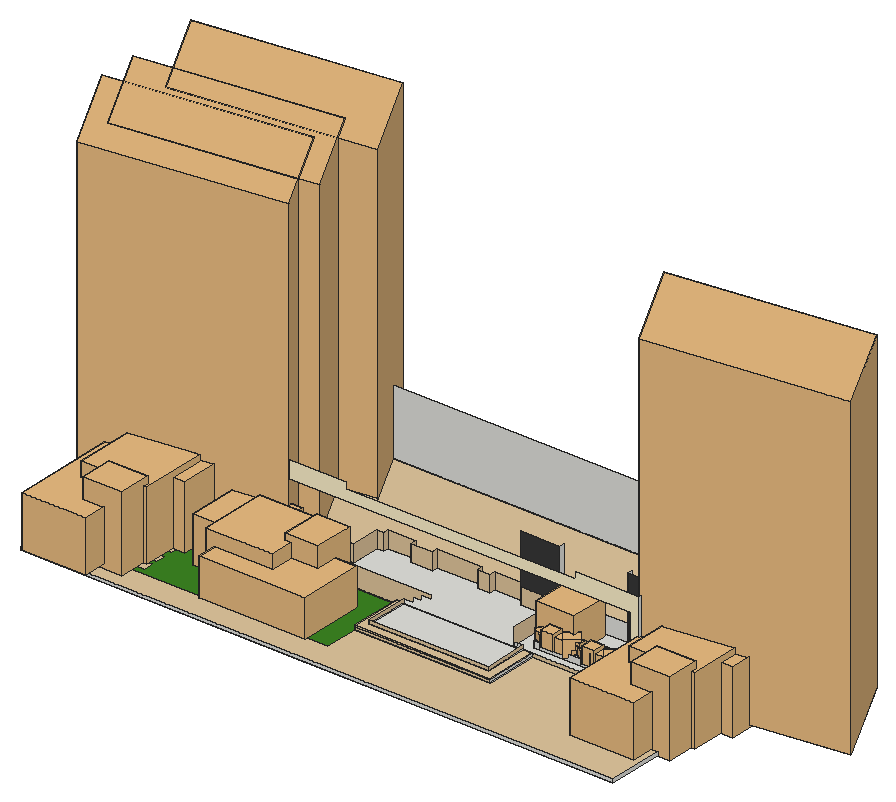
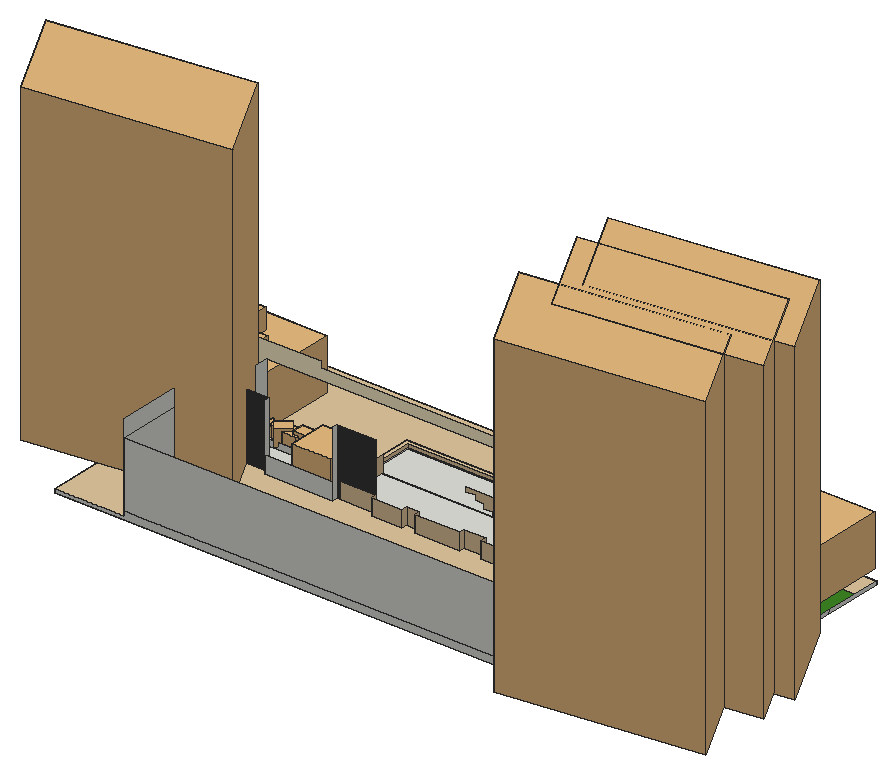
# SketchUp Ruby script. Lengths in inches.
U = 1.inch
M = Sketchup.active_model
def pt(a) = Geom::Point3d.new(a.map { |v| v * U })
def face(e, loops, mat)
  f = e.add_face(loops[0].map { |a| pt(a) })
  loops[1..].each { |l| e.add_face(l.map { |a| pt(a) }).erase! }
  f.material = f.back_material = mat if mat
  f
end
# faces: each face lists its corners as indices into pts; further lists are holes
def faces(e, pts, list, mat = nil) = list.each { |f| face(e, (f[0].is_a?(Array) ? f : [f]).map { |l| l.map { |i| pts[i] } }, mat) }
# xy, xz, yz: faces in a plane at the given z, y or x. An outline is a flat list of corners, or four numbers for a rectangle; further outlines are holes
def ring(l) = l.size == 4 ? [[l[0], l[1]], [l[2], l[1]], [l[2], l[3]], [l[0], l[3]]] : l.each_slice(2).to_a
def flat(e, list, mat, &to3) = list.each { |f| face(e, (f[0].is_a?(Array) ? f : [f]).map { |l| ring(l).map { |u, v| to3.(u, v) } }, mat) }
def xy(e, z, list, mat = nil) = flat(e, list, mat) { |x, y| [x, y, z] }
def xz(e, y, list, mat = nil) = flat(e, list, mat) { |x, z| [x, y, z] }
def yz(e, x, list, mat = nil) = flat(e, list, mat) { |y, z| [x, y, z] }
def lines(e, pts, list) = list.each { |a, b| e.add_line(pt(pts[a]), pt(pts[b])) }
# prism: a flat outline (further loops are holes) pulled along v
def prism(e, loops, v, mat = nil)
  f = face(e, loops, mat); d = Geom::Vector3d.new(v.map { |x| x * U })
  f.pushpull(f.normal.samedirection?(d) ? d.length : -d.length)
end
def box(e, o, s, mat = nil) = prism(e, [[o, [o[0] + s[0], o[1], o[2]], [o[0] + s[0], o[1] + s[1], o[2]], [o[0], o[1] + s[1], o[2]]]], [0, 0, s[2]], mat)
def at(x, y, z, deg = 0) = Geom::Transformation.translation(pt([x, y, z])) * Geom::Transformation.rotation(ORIGIN, Z_AXIS, deg.degrees)
def axes(o, x, y, z) = Geom::Transformation.new([*x, 0, *y, 0, *z, 0, *pt(o).to_a, 1])
def part(name) = M.definitions.add(name)
# library, detail: a bought-in or finely detailed component or shape, given as its bounding box
def library(name, o, s) = part(name).tap { |d| box(d.entities, o, s) }
def detail(e, o, s) = box(e.add_group.entities, o, s)
def put(e, d, t, mat = nil) = e.add_instance(d, t).tap { |i| i.material = mat if mat }
def group(e, t, mat = nil) = e.add_group.tap { |g| g.transformation = t; g.material = mat if mat }.entities
root = M.entities
M.materials.add("Material__1").color = [95, 70, 46]
M.materials.add("[Color A01]").color = [60, 133, 34]
M.materials.add("[Color D01]").color = [255, 242, 204]
M.materials.add("[Color M08]").color = [56, 56, 56]
M.materials.add("[Formica Beige]").color = [226, 199, 158]
c1 = library("Pot+Plant",[-20.81,-17.08,-0.03],[39.86,39.43,41.33])
c2 = library("Potted broadleaf plant",[-29.7,0,-10.87],[31.67,38.52,72.45])
c3 = part("Monstera_Pot_Quarter")
detail(c3.entities,[0.23,0.23,0],[9.32,9.32,13.9])
c4 = part("Monstera_Stem")
p = [[0.53,2.46,1.55],[0.55,2.41,0.71],[0.58,2.34,0.01],[0.58,2.59,0.01],[0.53,2.71,1.56],[0.48,2.66,3.11],
  [0.43,2.45,4.65],[0.38,2.07,6.15],[0.34,1.53,7.61],[0.29,0.84,9],[0.25,0,10.3125],[0.27,0.15,9.7],
  [0.3,0.62,8.89],[0.3,0.62,8.88],[0.34,1.3,7.51],[0.38,1.83,6.08],[0.43,2.2,4.6],[0.48,2.41,3.09],
  [0.53,2.46,1.5625],[0.33,2.59,0],[0.28,2.71,1.55],[0.23,2.66,3.1],[0.18,2.45,4.64],[0.13,2.07,6.15],
  [0.09,1.53,7.6],[0.04,0.84,8.99],[0,0,10.3]]
faces(c4.entities,p,[[0,1,2,3,4,5,6,7,8,9,10,11,12,13,14,15,16,17,18],[19,20,4,3],[20,21,5,4],[21,22,6,5],[22,23,7,6],[23,24,8,7],[24,25,9,8],[25,26,10,9]])
c5 = part("Monstera_Leaf_Half")
xy(c5.entities,0,[[9.39,-0.71,9.39,17.36,8.6,18.11,7.67,18.6875,6.64,19.0625,5.75,18.99,4.86,18.84,4,18.6,3.16,18.29,2.35,17.9,1.58,17.4375,0.86,16.91,0.33,15.95,0,14.91,0.64,15.5625,1.37,16.12,2.17,16.57,3.02,16.9,3.92,17.11,4.83,17.19,5.74,17.15,5.1,16.89,4.48,16.59,3.87,16.25,3.28,15.88,2.72,15.48,2.18,15.04,1.67,14.57,1.29,14.3,0.95,13.98,0.65,13.62,0.4,13.22,0.21,12.79,0.08,12.34,0.01,11.88,0.16,11.13,0.36,10.5,1.02,11.46,1.77,12.35,2.62,13.16,3.55,13.87,4.55,14.48,5.6,14.98,6.7,15.37,5.51,14.66,4.41,13.82,3.42,12.85,2.56,11.76,1.84,10.57,1.27,9.31,1.03,8.54,1.39,7.56,1.75,8.34,2.22,9.05,2.79,9.68,3.45,10.22,4.19,10.65,4.99,10.95,5.82,11.14,5.92,10.73,4.92,9.82,4.09,8.76,3.45,7.57,3.03,6.3,2.89,5.38,3.67,4.53,4.23,5.52,5,6.36,5.95,6.99,7.01,7.39,8.14,7.54,7.33,6.92,6.62,6.2,6,5.39,5.8125,4.66,5.76,3.92,5.83,3.17,6.03,2.45,7.95,4.19,6.73,2.06,6.96,1.71,7.24,1.375,7.55,1.08,7.89,0.8125,8.25,0.59,8.47,0.46,8.67,0.3125,8.86,0.14,9.03,-0.05,9.17,-0.26,9.29,-0.48]])
c6 = part("Monstera_Leaf_Half2")
xy(c6.entities,0,[[0,0,0.0625,0.14,0.14,0.28,0.23,0.41,0.33,0.53,0.44,0.64,0.57,0.73,0.7,0.8125,1.02,1.05,1.3125,1.33,1.58,1.63,0.92,3.26,1.66,1.76,1.8,1.96,2,2.31,1.99,2.65,1.9375,2.97,1.85,3.29,1.72,3.6,1.55,3.88,1.35,4.15,1.11,4.38,1.45,4.3,1.78,4.18,2.09,4.02,2.38,3.82,2.65,3.6,2.88,3.34,3.09,3.05,3.42,3.43,3.31,3.8125,3.15,4.18,2.96,4.54,2.74,4.87,2.48,5.18,2.19,5.46,1.88,5.7,1.88,6.2,2.29,6.15,2.68,6.02,3.05,5.83,3.38,5.58,3.67,5.27,3.89,4.93,4.06,4.54,4.28,4.99,4.17,5.67,3.98,6.32,3.7,6.94,3.34,7.52,2.9,8.04,2.4,8.51,2.18,8.66,2.18,8.85,2.46,8.8,3.05,8.58,3.57,8.25,4.02,7.82,4.37,7.3,4.61,6.73,4.72,6.12,5.05,6.79,4.86,7.39,4.6,7.96,4.26,8.49,3.85,8.97,3.39,9.4,2.87,9.75,2.3125,10.04,2.93,10.08,3.55,9.98,4.13,9.77,4.66,9.44,5.11,9,5.46,8.49,5.7,7.92,5.7,8.79,5.36,9.78,4.75,10.625,3.92,11.25,2.9375,11.6,1.9,11.65,0.89,11.39,0,10.84]])
c7 = part("Monstera_Leaf")
put(c7.entities,c5,axes([0,0.43,2.5],[0.6,0,0],[0,0.6,0],[0,0,1]))
put(c7.entities,c6,axes([5.63,0,2.5],[0.89879,0,-0.43837],[0,1,0],[0.43837,0,0.89879]))
c8 = part("Plant_Potted_Monstera")
g1 = group(c8.entities,at(-31.76,-2.48,0))
put(g1,c3,axes([41.19,13.38,0],[-1.05801,1.45623,0],[-1.45623,-1.05801,0],[0,0,1.8]))
put(g1,c3,axes([-4.47,6.15,0],[1.7119,-0.55623,0],[0.55623,1.7119,0],[0,0,1.8]))
put(g1,c3,axes([0,34.37,0],[0,-1.8,0],[1.8,0,0],[0,0,1.8]))
put(g1,c3,axes([28.22,38.84,0],[-1.7119,-0.55623,0],[0.55623,-1.7119,0],[0,0,1.8]))
put(g1,c3,axes([20.99,-6.82,0],[1.05801,1.45623,0],[-1.45623,1.05801,0],[0,0,1.8]))
g2 = group(c8.entities,at(-45.35,-10.84,22.35))
put(g2,c4,axes([31.57,11.47,0.05],[2.4,0,0],[0,2.4,0],[0,0,2.4]))
put(g2,c4,axes([37.07,37.75,-0.89],[-1.58858,0.45043,0.25253],[-0.40158,-1.59114,0.31185],[0.32464,0.23586,1.62148]))
put(g2,c4,axes([35.38,18.48,0],[3.25902,1.8816,0],[-2.0384,3.53061,0],[0,0,5.08031]))
put(g2,c4,axes([43.34,34.52,0.05],[-2.22411,3.85227,0],[-3.85227,-2.22411,0],[0,0,3.86995]))
put(g2,c4,axes([25.97,39.07,0.05],[-3.61063,-0.96747,0],[0.96747,-3.61063,0],[0,0,3.738]))
put(g2,c4,axes([21.76,18.96,0.05],[3.25939,-2.64884,0],[2.64884,3.25939,0],[0,0,4.2]))
put(g2,c4,axes([46.1,26.35,-0.74],[-0.50009,2.70618,0.3788],[-2.67394,-0.57497,0.46778],[0.59215,-0.31088,2.43223]))
put(g2,c4,axes([20.02,34.71,0.05],[-1.28976,-1.28976,0],[1.28976,-1.28976,0],[0,0,1.824]))
put(g2,c4,axes([15.69,19.9375,-0.89],[1.34133,-2.40299,0.42089],[2.34844,1.40191,0.51975],[-0.66056,0.10462,2.70247]))
put(g2,c7,axes([-0.47,22.84,6.14],[1.06874,-1.68333,0.43106],[0.69416,0.81107,1.44626],[-1.54881,-0.6934,1.13225]))
put(g2,c7,axes([50.87,17.94,4.27],[0.87503,1.76297,0.48288],[-0.72296,-0.14022,1.47584],[1.65009,-1.01401,0.5767]))
put(g2,c7,axes([49.79,39.97,-5.14],[-1.19278,1.56557,0.53653],[-0.62569,-0.953,1.38984],[1.49489,0.73546,1.17729]))
put(g2,c7,axes([50.65,23.15,27.2],[-0.38969,1.51702,-0.48773],[-0.81041,0.17386,1.24069],[1.35916,0.56845,0.81291]))
put(g2,c7,axes([26.42,52.09,4.7],[-1.67848,-1.12654,-0.48514],[0.50255,-1.2731,1.21752],[-1.0859,0.98249,1.47556]))
put(g2,c6,axes([32.94,54.6,23.93],[-1.59866,-0.5353,-1.42606],[-0.72066,-1.45568,1.3543],[-1.26669,1.65244,1.1021]))
put(g2,c5,axes([43.86,52.61,29.01],[-1.19529,0.14595,-0.47916],[-0.43239,-0.87341,0.81258],[-0.43769,1.71986,1.6157]))
put(g2,c6,axes([12.98,3.28,29],[2.16876,-0.96374,-0.35734],[0.84721,1.41614,1.32259],[-0.36343,-1.49947,1.83834]))
put(g2,c5,axes([3.26,12.46,26.83],[1.07397,-0.91411,0.29082],[0.50833,0.84969,0.79355],[-1.27737,-0.92524,1.80894]))
put(g2,c5,axes([30.81,4.39,33.875],[1.04828,0.47771,0],[-0.26309,0.57732,1.05032],[0.8619,-1.89133,1.14696]))
put(g2,c6,axes([40.84,8.47,33.13],[1.19248,1.54471,-0.50279],[-0.43849,0.96221,1.75054],[1.54056,-1.35089,1.03088]))
put(g2,c7,axes([26.17,-0.34,3.65],[1.93185,0,0.51764],[-0.36603,1.41421,1.36603],[-0.36603,-1.41421,1.36603]))
c9 = library("Plant+++Pot",[-21.48,-119.36,-205.6875],[86.44,86.43,89.41])
c10 = library("VEGETAÇÃO+TROPICAL+EM+VASOS",[-14.15,-83.94,15.25],[179.21,109.09,86.78])
c11 = part("Plant_Sago_Leaflet")
xy(c11.entities,0,[[3.85,0,0,3.85,0.11,3.95,1.79,2.46,3.89,0.03]])
c12 = part("Plant_Sago_Leaf_Half")
put(c12.entities,c11,axes([18.25,2.22,6.04],[-0.59922,0.82213,0.21597],[-0.84832,-0.5617,-0.21549],[0.05164,0.28878,-0.956]))
put(c12.entities,c11,axes([15.93,3.125,6.58],[0.84264,0.53805,0.02152],[0.5135,-0.79088,-0.33291],[0.1621,-0.29157,0.94271]))
put(c12.entities,c11,axes([17.26,3.125,6.23],[0.83553,0.54112,0.0953],[0.544,-0.79032,-0.2819],[0.07723,-0.28738,0.9547]))
put(c12.entities,c11,axes([21.85,2.14,5.59],[-0.54315,0.79051,0.28299],[-0.8361,-0.5401,-0.09604],[-0.07692,0.28878,-0.9543]))
put(c12.entities,c11,axes([16.82,3.14,6.36],[0.84574,0.52244,0.10852],[0.52878,-0.79337,-0.30158],[0.07147,-0.31244,0.94724]))
put(c12.entities,c11,axes([20.69,2.11,5.59],[-0.54315,0.79051,0.28299],[-0.8361,-0.5401,-0.09604],[-0.07692,0.28878,-0.9543]))
put(c12.entities,c11,axes([12.94,2.19,5.82],[-0.62836,0.82213,0.10425],[-0.79549,-0.5617,-0.36509],[0.22336,0.28878,-0.93098]))
put(c12.entities,c11,axes([5.63,1.77,3.66],[-0.51303,0.66403,-0.03839],[-0.55439,-0.45368,-0.43866],[0.4375,0.28878,-0.85159]))
put(c12.entities,c11,axes([1.66,2.73,2.01],[0.58222,0.45975,0.47335],[0.53533,-0.69817,0.01965],[-0.43842,-0.31244,0.84272]))
put(c12.entities,c11,axes([4.56,1.63,3.1],[-0.47333,0.61264,-0.03542],[-0.51149,-0.41858,-0.40472],[0.4375,0.28878,-0.85159]))
put(c12.entities,c11,axes([-0.77,2.08,0.33],[0.44115,0.36318,0.35932],[0.41167,-0.53384,0.03416],[-0.44824,-0.29157,0.84503]))
put(c12.entities,c11,axes([0.3125,2.32,0.91],[0.45211,0.40584,0.43976],[0.45211,-0.59274,0.08222],[-0.52272,-0.28738,0.80261]))
put(c12.entities,c11,axes([3.02,1.47,2.4],[-0.42197,0.55335,-0.07577],[-0.42197,-0.37807,-0.4111],[0.52272,0.28878,-0.80211]))
put(c12.entities,c11,axes([-0.06,2.25,0.73],[0.43704,0.37877,0.43722],[0.43704,-0.57519,0.06144],[-0.52272,-0.31244,0.79319]))
put(c12.entities,c11,axes([1.85,1.18,1.57],[-0.34089,0.44703,-0.06121],[-0.34089,-0.30543,-0.33211],[0.52272,0.28878,-0.80211]))
put(c12.entities,c11,axes([1.15,0.95,1.05],[-0.27036,0.35454,-0.04855],[-0.27036,-0.24223,-0.2634],[0.52272,0.28878,-0.80211]))
put(c12.entities,c11,axes([25.93,1.3,4.1875],[0.34606,0.16387,-0.04013],[0.13746,-0.32696,-0.14976],[0.25409,-0.31244,0.91532]))
put(c12.entities,c11,axes([27.16,1.16,3.94],[-0.26511,0.43857,0.21254],[-0.46539,-0.29965,0.03783],[-0.26081,0.28878,-0.92119]))
put(c12.entities,c11,axes([10.33,3.22,5.74],[0.84531,0.55957,0.23225],[0.60157,-0.82252,-0.2078],[-0.06911,-0.29157,0.95405]))
put(c12.entities,c11,axes([11.71,3.22,5.7],[0.81969,0.56277,0.30495],[0.61962,-0.82193,-0.14868],[-0.15438,-0.28738,0.94529]))
put(c12.entities,c11,axes([16.41,2.11,6.16],[-0.59523,0.79051,0.14422],[-0.78855,-0.5401,-0.29409],[0.15458,0.28878,-0.94483]))
put(c12.entities,c11,axes([11.35,3.11,5.7],[0.79491,0.52244,0.30851],[0.58575,-0.79337,-0.16572],[-0.15818,-0.31244,0.93667]))
put(c12.entities,c11,axes([15.42,2.11,6.03],[-0.59523,0.79051,0.14422],[-0.78855,-0.5401,-0.29409],[0.15458,0.28878,-0.94483]))
put(c12.entities,c11,axes([7.86,3.1,5.07],[0.79426,0.53805,0.28224],[0.59151,-0.79088,-0.1569],[-0.1388,-0.29157,0.94642]))
put(c12.entities,c11,axes([9.17,3.19,5.16],[0.78751,0.55736,0.36066],[0.6228,-0.81403,-0.10191],[-0.2232,-0.28738,0.93145]))
put(c12.entities,c11,axes([13.92,2.19,6.02],[-0.62836,0.82213,0.10425],[-0.79549,-0.5617,-0.36509],[0.22336,0.28878,-0.93098]))
put(c12.entities,c11,axes([8.78,3.11,5.14],[0.77018,0.52244,0.3659],[0.59631,-0.79337,-0.12238],[-0.22636,-0.31244,0.92257]))
put(c12.entities,c11,axes([18.75,2.9375,6.39],[0.79179,0.50576,-0.02955],[0.46209,-0.74343,-0.34263],[0.22098,-0.29157,0.93067]))
put(c12.entities,c11,axes([20.26,2.66,5.85],[0.71388,0.45995,0.03625],[0.44644,-0.67177,-0.26818],[0.13702,-0.28738,0.94797]))
put(c12.entities,c11,axes([24.12,1.9,5.09],[-0.46664,0.70355,0.28172],[-0.74803,-0.48069,-0.03859],[-0.13669,0.28878,-0.94759]))
put(c12.entities,c11,axes([19.74,2.79,6.05],[0.75729,0.46497,0.04913],[0.45283,-0.7061,-0.29743],[0.1308,-0.31244,0.94089]))
put(c12.entities,c11,axes([23.36,2.05,5.27],[-0.50334,0.75889,0.30388],[-0.80686,-0.5185,-0.04162],[-0.13669,0.28878,-0.94759]))
put(c12.entities,c11,axes([5.27,3.25,4.18],[0.79983,0.55957,0.35883],[0.62628,-0.82252,-0.11332],[-0.21425,-0.29157,0.93224]))
put(c12.entities,c11,axes([6.59,3.3125,4.37],[0.77807,0.57359,0.43497],[0.64728,-0.83774,-0.05314],[-0.29718,-0.28738,0.91055]))
put(c12.entities,c11,axes([11.36,2.24,5.62],[-0.6408,0.83003,0.05404],[-0.77099,-0.5671,-0.43182],[0.29731,0.28878,-0.91006]))
put(c12.entities,c11,axes([6.14,3.32,4.32],[0.78265,0.55379,0.45208],[0.64046,-0.84097,-0.07861],[-0.29962,-0.31244,0.90145]))
put(c12.entities,c11,axes([9.95,2.47,5.22],[-0.69674,0.71733,0],[-0.65281,-0.63408,-0.41447],[0.29731,0.28878,-0.91006]))
put(c12.entities,c11,axes([2.9,3.01,2.97],[0.70404,0.5219,0.41575],[0.59227,-0.76715,-0.03992],[-0.31683,-0.29157,0.90255]))
put(c12.entities,c11,axes([4.16,3.1,3.3125],[0.68371,0.54112,0.48961],[0.61243,-0.79032,0.01825],[-0.39682,-0.28738,0.87175]))
put(c12.entities,c11,axes([8.48,2.11,4.98],[-0.61222,0.79051,-0.01688],[-0.68385,-0.5401,-0.49055],[0.3969,0.28878,-0.87125]))
put(c12.entities,c11,axes([3.72,3.11,3.21],[0.68621,0.52244,0.50613],[0.60871,-0.79337,-0.00635],[-0.39823,-0.31244,0.86243]))
put(c12.entities,c11,axes([7.42,2,4.5],[-0.58161,0.75098,-0.01604],[-0.64966,-0.51309,-0.46602],[0.3969,0.28878,-0.87125]))
put(c12.entities,c11,axes([0.95,2.51,1.71],[0.5709,0.43582,0.37448],[0.4956,-0.64061,-0.01],[-0.359,-0.29157,0.88663]))
put(c12.entities,c11,axes([2.05,2.79,2.14],[0.5939,0.48701,0.46915],[0.5498,-0.71129,0.04237],[-0.43745,-0.28738,0.85209]))
put(c12.entities,c11,axes([21.85,2.26,5.91],[0.60131,0.38944,-0.10319],[0.31779,-0.57244,-0.30856],[0.34212,-0.29157,0.89327]))
put(c12.entities,c11,axes([23.3125,1.97,5.21],[0.52802,0.34091,-0.04335],[0.3017,-0.4979,-0.24078],[0.26119,-0.28738,0.92152]))
put(c12.entities,c11,axes([26.02,1.51,4.33],[-0.3385,0.56,0.27139],[-0.59423,-0.38261,0.0483],[-0.26081,0.28878,-0.92119]))
put(c12.entities,c11,axes([22.8125,2.09,5.46],[0.56785,0.34873,-0.0386],[0.30714,-0.52957,-0.26603],[0.25409,-0.31244,0.91532]))
put(c12.entities,c11,axes([25.32,1.67,4.61],[-0.37463,0.61976,0.30035],[-0.65765,-0.42344,0.05346],[-0.26081,0.28878,-0.92119]))
put(c12.entities,c11,axes([24.85,1.53,4.8],[0.41289,0.26741,-0.07085],[0.21821,-0.39307,-0.21188],[0.34212,-0.29157,0.89327]))
put(c12.entities,c11,axes([26.68,0.99,3.82],[0.25671,0.06521,-0.05243],[0.04503,-0.25025,-0.0908],[0.26119,-0.28738,0.92152]))
put(c12.entities,c11,axes([27.77,0.93,3.67],[-0.21503,0.35573,0.1724],[-0.37748,-0.24304,0.03068],[-0.26081,0.28878,-0.92119]))
put(c12.entities,c11,axes([13.12,3.125,6.23],[0.83216,0.53805,0.13423],[0.55347,-0.79088,-0.26111],[0.03433,-0.29157,0.95593]))
put(c12.entities,c11,axes([14.42,3.22,6.08],[0.83968,0.55736,0.21258],[0.59417,-0.81403,-0.21266],[-0.05138,-0.28738,0.95644]))
put(c12.entities,c11,axes([19.12,2.14,6.04],[-0.57617,0.79051,0.20766],[-0.8157,-0.5401,-0.2072],[0.05164,0.28878,-0.956]))
put(c12.entities,c11,axes([14.04,3.14,6.125],[0.82358,0.52244,0.22086],[0.56442,-0.79337,-0.22802],[-0.0561,-0.31244,0.94828]))
c13 = part("Plant_Sago_Leaf")
p = [[20.17,5.46,5.15],[23.14,5.46,4.71],[14.17,5.46,5.15],[17.17,5.46,5.3],[26.05,5.46,3.96],[27.46,5.46,3.45],
  [8.29,5.46,3.96],[11.2,5.46,4.71],[0.2,5.46,0.05],[2.76,5.46,1.625],[5.47,5.46,2.93],[-1.21,5.46,-2.04],
  [-1.11,5.46,-1.51],[-0.4,5.46,-0.47]]
lines(c13.entities,p,[[0,1],[2,3],[3,0],[1,4],[4,5],[6,7],[7,2],[8,9],[9,10],[10,6],[11,12],[13,8],
  [12,13]])
put(c13.entities,c12,axes([0.55,5.52,0.34],[0.99974,0,-0.02269],[0,-1,0],[0.02269,0,0.99974]))
put(c13.entities,c12,at(0,5.37,0))
c14 = part("Plant_Sago_Stem")
xy(c14.entities,4.5,[[2.49,1.71,3.51,1.71,4.03,2.6,3.51,3.49,2.49,3.49,1.97,2.6]])
p = [[1.74,0.42,2],[0.48,2.6,2],[0,2.6,0],[1.5,0,0],[4.5,0,0],[4.26,0.42,2],
  [6,2.6,0],[5.52,2.6,2],[1.74,4.78,2],[1.5,5.2,0],[4.5,5.2,0],[4.26,4.78,2],
  [2.16,1.14,3.5],[1.3125,2.6,3.5],[3.84,1.14,3.5],[4.6875,2.6,3.5],[2.16,4.06,3.5],[3.84,4.06,3.5],
  [2.49,1.71,4.5],[1.97,2.6,4.5],[3.51,1.71,4.5],[4.03,2.6,4.5],[2.49,3.49,4.5],[3.51,3.49,4.5]]
faces(c14.entities,p,[[0,1,2,3],[4,5,0,3],[4,6,7,5],[1,8,9,2],[6,10,11,7],[9,8,11,10],[12,13,1,0],[5,14,12,0],
  [5,7,15,14],[13,16,8,1],[7,11,17,15],[8,16,17,11],[18,19,13,12],[14,20,18,12],[14,15,21,20],[19,22,16,13],
  [15,17,23,21],[16,22,23,17]])
c15 = part("sketchup-download200609201909046")
put(c15.entities,c13,axes([-0.61,6.35,3.08],[-0.3501,0.13195,-0.09971],[-0.32249,-0.79038,0.08641],[-0.20289,0.18785,0.96101]))
put(c15.entities,c13,axes([-2.8125,-4.7,5],[0.405,-0.70148,0],[0.6755,0.39,0],[0,0,1]))
put(c15.entities,c13,axes([1.31,-3,6.53],[0.51791,0.17354,0.20258],[-0.22103,0.74449,-0.07268],[-0.35965,-0.0157,0.93295]))
put(c15.entities,c13,axes([-3.58,0.28,6.65],[-0.14067,-0.52499,0.20972],[0.75342,-0.20188,0],[0.09317,0.34773,0.93295]))
put(c15.entities,c13,axes([2.47,4.23,5.54],[-0.305,0.52828,0],[-0.6755,-0.39,0],[0,0,1]))
put(c15.entities,c13,axes([-2.48,4.68,4.96],[-0.74801,0,0.20043],[0,-0.858,0],[0.25882,0,0.96593]))
put(c15.entities,c14,at(-3,-2.6,0))
put(c15.entities,c13,axes([4.98,0.12,5.54],[0.375,0.64952,0],[-0.6755,0.39,0],[0,0,1]))
put(c15.entities,c13,axes([-5.18,-1.3,3.84],[-0.32872,-0.56937,-0.13256],[0.60795,-0.351,0],[-0.09883,-0.17118,0.98027]))
put(c15.entities,c13,axes([1.82,3.73,6.67],[-0.37415,0.09357,0.38234],[-0.24005,-0.683,-0.06775],[0.60151,-0.27651,0.6563]))
put(c15.entities,c13,axes([3.71,-4.26,4.17],[0.48705,0,-0.2812],[0,0.78,0],[0.5,0,0.86603]))
c16 = part("Untitled (12)")
put(c16.entities,c15,axes([8.31,12.62,2.43],[2.68,0,0],[0,2.68,0],[0,0,2.68]))
c17 = library("Palm tree",[-4.09,-4.52,0],[193.52,193.51,258.93])
c18 = part("Palm+Tree")
put(c18.entities,c17,at(25.51,-21.81,0,15))
c19 = library("Areca palm plant",[0,0,0],[49.1,36.6,54.46])
c20 = library("Group\#6",[-84.69,-90.07,-0.36],[176.51,175.13,171.4])
c21 = library("Group20\#1",[-20.81,-17.08,3.79],[39.86,39.43,37.51])
c22 = library("Group\#130",[-7.34,-1.2,0],[38.67,35.81,49.04])
c23 = library("Group38\#2",[14.01,28.44,-23.43],[18.58,18.32,38.89])
xy(root,-8.375,[[0,0,704.82,145.8125],[704.82,0,1037.26,145.8125],[1037.26,0,1456.54,145.8125],[0,145.8125,704.82,274.5],[704.82,145.8125,704.82,274.5,0,274.5,0,701.99,1456.54,701.99,1456.54,274.5,1037.26,274.5,1037.26,145.8125],
  [1037.26,145.8125,1456.54,274.5]])
xy(root,0,[[1264.2,290.49,1286.86,406.8125]])
xy(root,0,[[[0,64.5,703.93,64.5,704.82,145.8125,704.82,274.5,0,274.5],[214.21,115.32,243.02,144.13],[214.21,160.25,243.02,189.07],[214.21,199.5,243.02,228.32],[214.21,243.5,243.02,272.32],[214.21,77.5,243.02,106.32]]],"[Color A01]")
xy(root,0,[[0,0,1456.54,0,1456.54,701.99,1286.86,701.99,1286.86,274.5,1037.26,274.5,1037.26,145.8125,704.82,145.8125,703.93,64.5,0,64.5],[214.21,77.5,243.02,106.32],[214.21,115.32,243.02,144.13],[214.21,160.25,243.02,189.07],[214.21,199.5,243.02,228.32],
  [214.21,243.5,243.02,272.32]],"[Formica Beige]")
xy(root,6.92,[[704.82,145.8125,1037.26,274.5]],"[Formica Beige]")
xy(root,7.44,[[722.74,167.6875,1015.74,274.5]])
xy(root,10,[[991.92,274.5,1286.86,274.5,1286.86,290.49,1264.2,290.49,1264.2,406.8125,1165.59,406.8125,1165.59,420.5625,999.61,420.5625,999.61,406.8125,991.92,406.8125],[1264.2,290.49,1286.86,406.8125],[0,336.9375,204.29,701.99]])
xy(root,10,[[704.82,145.8125,1037.26,145.8125,1037.26,274.5,1015.74,274.5,1015.74,167.6875,722.74,167.6875,722.74,274.5,704.82,274.5],[204.29,336.9375,263.51,336.9375,263.51,347.22,504.95,347.22,504.95,336.9375,549.32,336.9375,549.32,406.8125,566.51,406.8125,566.51,420.5625,633.8,420.5625,633.8,406.8125,687.15,406.8125,687.15,420.5625,797.18,420.5625,797.18,406.8125,828.83,406.8125,828.83,420.5625,903,420.5625,903,406.8125,999.61,406.8125,999.61,420.5625,1165.59,420.5625,1165.59,406.8125,1286.86,406.8125,1286.86,701.99,204.29,701.99]],"[Formica Beige]")
xz(root,0,[[0,-8.375,1456.54,0]])
xz(root,145.8125,[[704.82,-8.375,1037.26,0]])
xz(root,145.8125,[[704.82,0,1037.26,6.92],[704.82,6.92,1037.26,10]],"[Formica Beige]")
xz(root,167.6875,[[722.74,7.44,1015.74,10],[722.74,10,1015.74,18.94]],"[Formica Beige]")
xz(root,274.5,[[0,-8.375,704.82,0],[991.92,10,1000.23,18.94],[1000.23,10,1015.74,18.94]])
xz(root,274.5,[[0,0,704.82,0,704.82,10,722.74,10,722.74,18.94,744.1,18.94,744.1,29.9,763.95,29.9,763.95,40.875,787.73,40.875,787.73,50.65,0,50.65],[1037.26,0,1286.86,10],[704.82,6.92,1037.26,6.92,1037.26,10,1015.74,10,1015.74,7.44,722.74,7.44,722.74,10,704.82,10]],"[Formica Beige]")
xz(root,290.49,[[1264.2,10,1286.86,10,1286.86,213.5625,1132.55,213.5625,1132.55,198,566.56,198,566.56,213.5625,204.29,213.5625,204.29,172.0625,1264.2,172.0625]],"[Color D01]")
xz(root,290.49,[[1264.2,0,1286.86,10]],"[Formica Beige]")
xz(root,336.9375,[[0,10,204.29,50.65]])
xz(root,336.9375,[[204.29,10,263.51,50.65],[504.95,10,549.32,50.65]],"[Formica Beige]")
xz(root,347.22,[[263.51,10,504.95,50.65]],"[Formica Beige]")
xz(root,406.8125,[[1264.2,0,1286.86,10],[1264.2,10,1286.86,172.0625]])
xz(root,406.8125,[[991.92,10,999.61,10,999.61,172.0625,903,172.0625,903,50.65,991.92,50.65],[1165.59,10,1264.2,172.0625]],"[Color M08]")
xz(root,406.8125,[[549.32,10,566.51,50.65],[633.8,10,687.15,50.65],[797.18,10,828.83,50.65],[903,10,991.92,50.65]],"[Formica Beige]")
xz(root,420.5625,[[999.61,10,1165.59,52.0625]])
xz(root,420.5625,[[566.51,10,633.8,50.65],[687.15,10,797.18,50.65],[828.83,10,903,50.65]],"[Formica Beige]")
xz(root,701.99,[[0,-8.375,0,10,1286.86,10,1286.86,0,1456.54,0,1456.54,-8.375],[204.29,10,1286.86,172.0625]])
yz(root,0,[[0,-8.375,145.8125,0],[145.8125,-8.375,274.5,0],[274.5,-8.375,274.5,50.65,336.9375,50.65,336.9375,10,701.99,10,701.99,-8.375]])
yz(root,204.29,[[336.9375,10,701.99,172.0625]],"[Formica Beige]")
yz(root,263.51,[[336.9375,10,347.22,50.65]],"[Formica Beige]")
yz(root,504.95,[[336.9375,10,347.22,50.65]],"[Formica Beige]")
yz(root,549.32,[[336.9375,10,406.8125,50.65]],"[Formica Beige]")
yz(root,566.51,[[406.8125,10,420.5625,50.65]],"[Formica Beige]")
yz(root,633.8,[[406.8125,10,420.5625,50.65]],"[Formica Beige]")
yz(root,687.15,[[406.8125,10,420.5625,50.65]],"[Formica Beige]")
yz(root,704.82,[[145.8125,-8.375,274.5,0],[145.8125,0,274.5,6.92]])
yz(root,704.82,[[145.8125,6.92,274.5,10]],"[Formica Beige]")
yz(root,722.74,[[167.6875,7.44,274.5,10]])
yz(root,722.74,[[167.6875,10,274.5,18.94]],"[Formica Beige]")
yz(root,797.18,[[406.8125,10,420.5625,50.65]],"[Formica Beige]")
yz(root,828.83,[[406.8125,10,420.5625,50.65]],"[Formica Beige]")
yz(root,903,[[406.8125,10,420.5625,50.65]],"[Formica Beige]")
yz(root,991.92,[[274.5,10,406.8125,50.65]],"[Formica Beige]")
yz(root,999.61,[[406.8125,10,420.5625,172.0625]])
yz(root,1015.74,[[167.6875,7.44,274.5,10]])
yz(root,1015.74,[[167.6875,10,274.5,18.94]],"[Formica Beige]")
yz(root,1037.26,[[145.8125,-8.375,274.5,0],[145.8125,0,274.5,6.92]])
yz(root,1037.26,[[145.8125,6.92,274.5,10]],"[Formica Beige]")
yz(root,1165.59,[[406.8125,10,420.5625,172.0625]])
yz(root,1264.2,[[290.49,10,406.8125,172.0625]])
yz(root,1264.2,[[290.49,0,406.8125,10]],"[Formica Beige]")
yz(root,1286.86,[[274.5,0,290.49,10],[290.49,0,406.8125,10],[290.49,10,406.8125,10,406.8125,172.0625,701.99,172.0625,701.99,213.5625,290.49,213.5625],[406.8125,10,701.99,172.0625]])
yz(root,1286.86,[[406.8125,0,701.99,10]],"[Formica Beige]")
yz(root,1456.54,[[0,-8.375,145.8125,0],[145.8125,-8.375,274.5,0],[274.5,-8.375,701.99,0]])
put(root,c1,axes([381.09,216.45,-44.78],[3.7846,0,0],[0,3.7846,0],[0,0,3.7846]))
put(root,c2,axes([593.16,165.02,-17.28],[2.53568,0,0],[0,2.53568,0],[0,0,2.53568]))
put(root,c8,axes([508.01,174.84,-44.84],[1.8923,0,0],[0,1.8923,0],[0,0,1.8923]))
put(root,c9,axes([410.34,334.14,344.375],[1.8923,0,0],[0,1.8923,0],[0,0,1.8923]))
put(root,c10,axes([412.55,180.6,-57.61],[1.45,0,0],[0,1.45,0],[0,0,1.45]))
put(root,c16,at(362.82,178.21,0))
put(root,c1,axes([1440.61,353.71,-9.29],[0,-3.7846,0],[3.7846,0,0],[0,0,3.7846]))
put(root,c2,axes([1389.18,141.64,18.21],[0,-2.53568,0],[2.53568,0,0],[0,0,2.53568]))
put(root,c9,axes([1558.3,324.46,379.87],[0,-1.8923,0],[1.8923,0,0],[0,0,1.8923]))
put(root,c1,axes([1059.92,359.11,-2.65],[2.37,0,0],[0,2.37,0],[0,0,2.37]))
put(root,c18,axes([1224.375,330.75,0],[2.52,0,0],[0,1.26,0],[0,0,2.9988]))
put(root,c18,axes([-100.18,355.67,0],[2.52,0,0],[0,1.26,0],[0,0,2.9988]))
put(root,c18,axes([-100.18,533.86,0],[2.52,0,0],[0,1.26,0],[0,0,2.9988]))
put(root,c18,axes([-100.18,260.05,0],[2.52,0,0],[0,1.26,0],[0,0,2.9988]))
put(root,c10,axes([1404.75,322.26,-22.11],[0,-1.45,0],[1.45,0,0],[0,0,1.45]))
put(root,c1,axes([178.24,248.9375,0.54],[0,-3.7846,0],[3.7846,0,0],[0,0,3.7846]))
put(root,c2,axes([126.81,36.87,28.05],[0,-2.53568,0],[2.53568,0,0],[0,0,2.53568]))
put(root,c9,axes([295.93,219.6875,389.7],[0,-1.8923,0],[1.8923,0,0],[0,0,1.8923]))
put(root,c10,axes([142.38,217.48,-12.28],[0,-1.45,0],[1.45,0,0],[0,0,1.45]))
g3 = group(root,at(1261.66,292.73,10,90))
put(g3,c19,axes([-6.2,56.6,6.08],[0.45017,-0.56191,0],[0.66137,0.52986,0],[0,0,0.72]))
put(g3,c19,axes([-6.2,158.41,6.08],[0.45017,-0.56191,0],[0.66137,0.52986,0],[0,0,0.72]))
put(g3,c20,axes([17.19,223.04,6.07],[-0.08133,-0.14087,0],[0.14087,-0.08133,0],[0,0,0.1725]))
put(g3,c20,axes([14.93,44.05,6.05],[-0.04961,-0.08593,0],[0.08593,-0.04961,0],[0,0,0.10522]))
put(g3,c21,axes([18.97,79.98,4.77],[0,0.85,0],[-0.85,0,0],[0,0,0.85]))
put(g3,c20,axes([17.19,121.23,6.07],[-0.08133,-0.14087,0],[0.14087,-0.08133,0],[0,0,0.1725]))
put(g3,c20,axes([14.93,91.37,6.05],[-0.04961,-0.08593,0],[0.08593,-0.04961,0],[0,0,0.10522]))
put(g3,c20,axes([14.93,145.87,6.05],[-0.04961,-0.08593,0],[0.08593,-0.04961,0],[0,0,0.10522]))
put(g3,c20,axes([14.93,173.12,6.05],[-0.04961,-0.08593,0],[0.08593,-0.04961,0],[0,0,0.10522]))
put(g3,c22,axes([24.9375,89.91,8],[0,0.79,0],[-0.79,0,0],[0,0,0.79]))
put(g3,c23,axes([-4.1,-1.15,28.17],[0.8848,0,0],[0,0.94674,0],[0,0,0.85826]))
put(g3,c20,axes([14.93,71.3,6.05],[-0.04961,-0.08593,0],[0.08593,-0.04961,0],[0,0,0.10522]))
put(g3,c20,axes([14.93,193.18,6.05],[-0.04961,-0.08593,0],[0.08593,-0.04961,0],[0,0,0.10522]))
put(g3,c20,axes([17.19,15.79,6.07],[-0.08133,-0.14087,0],[0.14087,-0.08133,0],[0,0,0.1725]))
put(g3,c22,axes([24.9375,191.72,8],[0,0.79,0],[-0.79,0,0],[0,0,0.79]))
put(g3,c21,axes([18.97,181.79,4.77],[0,0.85,0],[-0.85,0,0],[0,0,0.85]))
g4 = group(g3,at(0,0,0))
xy(g4,0,[[0,0,6,234.8],[30,0,36,234.8]])
xy(g4,3,[[6,0,30,234.8]])
xy(g4,7,[[6,5,30,229.8]],"Material__1")
xy(g4,15,[[[0,0,36,234.8],[6,5,30,229.8]]])
xz(g4,0,[[0,0,6,0,6,3,30,3,30,0,36,0,36,15,0,15]])
xz(g4,5,[[6,7,30,15]])
xz(g4,229.8,[[6,7,30,15]])
xz(g4,234.8,[[0,0,0,15,36,15,36,0,30,0,30,3,6,3,6,0]])
yz(g4,0,[[0,0,234.8,15]])
yz(g4,6,[[0,0,234.8,3],[5,7,229.8,15]])
yz(g4,30,[[0,0,234.8,3],[5,7,229.8,15]])
yz(g4,36,[[0,0,234.8,15]])
put(g3,c23,axes([-4.1,100.66,28.17],[0.8848,0,0],[0,0.94674,0],[0,0,0.85826]))
